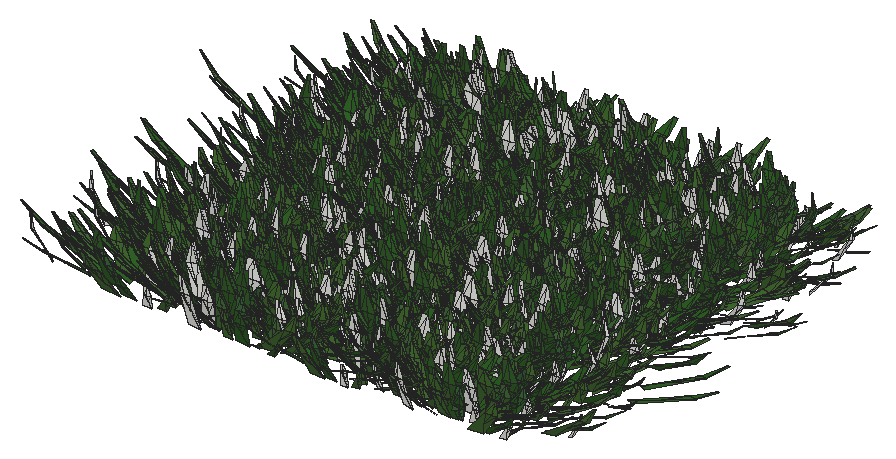
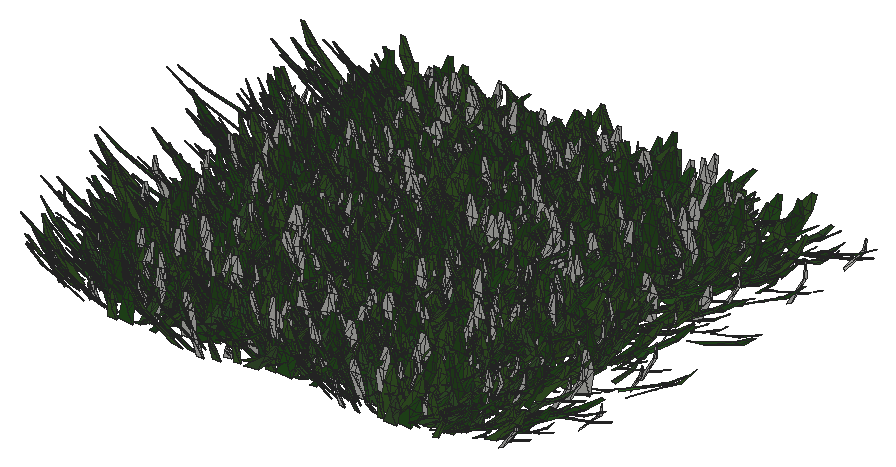
# SketchUp Ruby script. Lengths in inches.
U = 1.inch
M = Sketchup.active_model
def pt(a) = Geom::Point3d.new(a.map { |v| v * U })
def face(e, loops, mat)
  f = e.add_face(loops[0].map { |a| pt(a) })
  loops[1..].each { |l| e.add_face(l.map { |a| pt(a) }).erase! }
  f.material = f.back_material = mat if mat
  f
end
# faces: each face lists its corners as indices into pts; further lists are holes
def faces(e, pts, list, mat = nil) = list.each { |f| face(e, (f[0].is_a?(Array) ? f : [f]).map { |l| l.map { |i| pts[i] } }, mat) }
# xy, xz, yz: faces in a plane at the given z, y or x. An outline is a flat list of corners, or four numbers for a rectangle; further outlines are holes
def ring(l) = l.size == 4 ? [[l[0], l[1]], [l[2], l[1]], [l[2], l[3]], [l[0], l[3]]] : l.each_slice(2).to_a
def flat(e, list, mat, &to3) = list.each { |f| face(e, (f[0].is_a?(Array) ? f : [f]).map { |l| ring(l).map { |u, v| to3.(u, v) } }, mat) }
def xy(e, z, list, mat = nil) = flat(e, list, mat) { |x, y| [x, y, z] }
def xz(e, y, list, mat = nil) = flat(e, list, mat) { |x, z| [x, y, z] }
def yz(e, x, list, mat = nil) = flat(e, list, mat) { |y, z| [x, y, z] }
def lines(e, pts, list) = list.each { |a, b| e.add_line(pt(pts[a]), pt(pts[b])) }
# prism: a flat outline (further loops are holes) pulled along v
def prism(e, loops, v, mat = nil)
  f = face(e, loops, mat); d = Geom::Vector3d.new(v.map { |x| x * U })
  f.pushpull(f.normal.samedirection?(d) ? d.length : -d.length)
end
def box(e, o, s, mat = nil) = prism(e, [[o, [o[0] + s[0], o[1], o[2]], [o[0] + s[0], o[1] + s[1], o[2]], [o[0], o[1] + s[1], o[2]]]], [0, 0, s[2]], mat)
def at(x, y, z, deg = 0) = Geom::Transformation.translation(pt([x, y, z])) * Geom::Transformation.rotation(ORIGIN, Z_AXIS, deg.degrees)
def axes(o, x, y, z) = Geom::Transformation.new([*x, 0, *y, 0, *z, 0, *pt(o).to_a, 1])
def part(name) = M.definitions.add(name)
# library, detail: a bought-in or finely detailed component or shape, given as its bounding box
def library(name, o, s) = part(name).tap { |d| box(d.entities, o, s) }
def detail(e, o, s) = box(e.add_group.entities, o, s)
def put(e, d, t, mat = nil) = e.add_instance(d, t).tap { |i| i.material = mat if mat }
def group(e, t, mat = nil) = e.add_group.tap { |g| g.transformation = t; g.material = mat if mat }.entities
root = M.entities
M.materials.add("Material10").color = [48, 100, 38]
M.materials.add("Material3").color = [68, 110, 58]
M.materials.add("Material4").color = [48, 90, 38]
M.materials.add("Material5").color = [68, 110, 48]
M.materials.add("Material6").color = [48, 90, 48]
M.materials.add("Material7").color = [58, 110, 58]
M.materials.add("Material8").color = [58, 90, 38]
M.materials.add("Material9").color = [68, 100, 58]
c1 = part("grass00")
p = [[-0.6875,0.15,0],[-0.56,0.08,5.52],[-0.04,0.03,2.76],[0.48,-0.02,0],[0.35,-0.02,5.52],[-0.1,-0.14,5.52],
  [-0.12,0.65,8.37],[-0.42,0.65,8.37]]
faces(c1.entities,p,[[0,1,2,3],[3,2,4],[1,5,2],[5,4,2],[1,6,5],[4,5,6],[7,6,1]])
c2 = part("Group16\#1")
put(c2.entities,c1,axes([1.44,-0.61,-0.01],[0.05352,0.12609,0],[-0.10704,0.04543,0.07239],[0.06664,-0.02828,0.11628]),"Material6")
put(c2.entities,c1,axes([0.76,-0.15,-0.01],[0.04676,0.24062,0],[-0.23162,0.04501,0.06642],[0.0652,-0.01267,0.23595]),"Material3")
put(c2.entities,c1,axes([0.79,0.01,-0.01],[-0.00606,0.34651,0],[-0.34381,-0.00602,0.0432],[0.04319,0.00076,0.34386]))
put(c2.entities,c1,axes([1,0.23,-0.01],[-0.07192,0.31144,0],[-0.28722,-0.06632,0.1236],[0.12043,0.02781,0.29478]),"Material5")
put(c2.entities,c1,axes([1.66,0.77,-0.01],[-0.13828,0.29651,0],[-0.21551,-0.1005,0.22471],[0.20365,0.09498,0.23779]),"Material10")
put(c2.entities,c1,axes([0.6875,0.52,-0.01],[-0.18126,0.24051,0],[-0.22746,-0.17142,0.09788],[0.07817,0.05891,0.28481]),"Material5")
put(c2.entities,c1,axes([0.68,0.78,-0.01],[-0.215,0.18688,0],[-0.12385,-0.14248,0.21334],[0.13995,0.16101,0.18878]),"Material3")
put(c2.entities,c1,axes([0.56,1,-0.01],[-0.13756,0.07624,0],[-0.06159,-0.11112,0.0927],[0.04494,0.08108,0.12705]),"Material5")
put(c2.entities,c1,axes([0.2,0.64,-0.01],[-0.23729,0.07254,0],[-0.05711,-0.18681,0.153],[0.04473,0.14632,0.19535]),"Material10")
put(c2.entities,c1,axes([0.0625,0.72,-0.01],[-0.28874,0.02525,0],[-0.02179,-0.24916,0.14647],[0.01276,0.14591,0.25012]),"Material3")
put(c2.entities,c1,axes([-0.08,0.62,-0.01],[-0.34089,-0.04187,0],[0.03255,-0.26504,0.216],[-0.02633,0.21439,0.26703]),"Material10")
put(c2.entities,c1,axes([-0.34,0.98,-0.01],[-0.14314,-0.0493,0],[0.04397,-0.12769,0.06843],[-0.02228,0.0647,0.13505]),"Material10")
put(c2.entities,c1,axes([-0.87,1.45,-0.01],[-0.23488,-0.14114,0],[0.13761,-0.22901,0.06087],[-0.03135,0.05217,0.26717]))
put(c2.entities,c1,axes([-0.72,0.77,-0.01],[-0.14208,-0.13251,0],[0.07209,-0.0773,0.16301],[-0.11118,0.11922,0.1057]),"Material10")
put(c2.entities,c1,axes([-0.62,0.43,-0.01],[-0.14845,-0.21203,0],[0.18654,-0.13061,0.12304],[-0.10079,0.07057,0.22772]),"Material3")
put(c2.entities,c1,axes([-0.68,0.29,-0.01],[-0.13639,-0.32136,0],[0.31723,-0.13464,0.05579],[-0.05136,0.0218,0.34462]),"Material4")
put(c2.entities,c1,axes([-0.64,0.125,-0.01],[-0.0458,-0.23569,0],[0.22124,-0.043,0.08276],[-0.08124,0.01579,0.22538]),"Material7")
put(c2.entities,c1,axes([-1.6,-0.03,-0.01],[0.00576,-0.32897,0],[0.27526,0.00482,0.18018],[-0.18015,-0.00315,0.2753]),"Material5")
put(c2.entities,c1,axes([-1.36,-0.31,-0.01],[0.05718,-0.24765,0],[0.18172,0.04196,0.17267],[-0.16825,-0.03885,0.1865]),"Material10")
put(c2.entities,c1,axes([-1.54,-0.72,-0.01],[0.06537,-0.14017,0],[0.13555,0.06321,0.03939],[-0.0357,-0.01665,0.14956]))
put(c2.entities,c1,axes([-1.19,-0.9,-0.01],[0.09597,-0.12735,0],[0.11214,0.08451,0.07557],[-0.06035,-0.04548,0.14042]),"Material9")
put(c2.entities,c1,axes([-0.47,-0.54,-0.01],[0.11588,-0.10072,0],[0.0618,0.0711,0.12124],[-0.07953,-0.0915,0.0942]))
put(c2.entities,c1,axes([-0.47,-0.84,-0.01],[0.11927,-0.0661,0],[0.06603,0.11913,0.00646],[-0.00313,-0.00565,0.13621]),"Material5")
put(c2.entities,c1,axes([-0.38,-1.24,-0.01],[0.28037,-0.08571,0],[0.0618,0.20215,0.20315],[-0.05939,-0.19428,0.21139]),"Material9")
put(c2.entities,c1,axes([-0.06,-0.66,-0.01],[0.22719,-0.01987,0],[0.01247,0.14255,0.17758],[-0.01547,-0.17691,0.1431]),"Material8")
put(c2.entities,c1,axes([0.11,-0.89,-0.01],[0.14882,0.01828,0],[-0.01058,0.08611,0.12229],[0.01491,-0.12138,0.08676]),"Material6")
put(c2.entities,c1,axes([0.25,-0.72,-0.01],[0.20481,0.07053,0],[-0.06206,0.18022,0.10291],[0.03351,-0.0973,0.1906]),"Material6")
put(c2.entities,c1,axes([0.85,-1.42,-0.01],[0.16481,0.09904,0],[-0.09472,0.15762,0.05616],[0.02893,-0.04814,0.18389]),"Material5")
put(c2.entities,c1,axes([1.01,-1.09,-0.01],[0.21858,0.20385,0],[-0.17495,0.1876,0.15339],[0.10462,-0.11218,0.25652]),"Material10")
put(c2.entities,c1,axes([1.01,-0.71,-0.01],[0.08733,0.12473,0],[-0.06445,0.04512,0.13037],[0.1068,-0.07477,0.07867]),"Material6")
c3 = part("Group15\#1")
put(c3.entities,c2,at(0,0,0))
c4 = part("3darcstudiotree_grass00\#1")
put(c4.entities,c3,at(0,0,0))
put(root,c4,axes([993.125,915.59,0],[-3.60582,-0.24196,0],[1.04886,-0.97693,-0.03217],[0.06139,-0.05718,1.86146]))
put(root,c4,axes([991.19,900.47,0],[2.28978,0.96186,0],[-3.76338,0.55994,-0.00188],[-0.01111,0.00165,1.87843]))
put(root,c4,axes([991.63,916.75,0],[2.13866,0.74246,0],[-3.14038,0.56537,-0.02117],[-0.12042,0.02168,1.69559]))
put(root,c4,axes([992.37,908.81,0],[-2.16053,0.9205,0],[-4.3515,-0.63835,-0.01374],[-0.05636,-0.00827,1.50009]))
put(root,c4,axes([991.97,894.3,0],[0.82896,1.15167,0],[-5.08245,0.22864,-0.03105],[-0.14233,0.0064,1.50318]))
put(root,c4,axes([992.18,919.85,0],[4.96916,0.09392,0],[-0.36542,1.20834,-0.04634],[-0.02294,0.07584,1.98901]))
put(root,c4,axes([992.33,926.2,0],[1.48031,1.01744,0],[-4.79783,0.43628,-0.0524],[-0.2112,0.01921,1.36852]))
put(root,c4,axes([994.4,929.09,0],[-4.63446,-0.46393,0],[1.56749,-0.97866,-0.04264],[0.10164,-0.06346,1.69007]))
put(root,c4,axes([993.33,930.77,0],[3.16295,-0.50135,0],[2.10496,0.83,-0.03299],[0.1278,0.05039,1.77748]))
put(root,c4,axes([993.96,903.53,0],[-3.25579,0.4273,0],[-2.23495,-1.06431,-0.02543],[-0.07509,-0.03576,1.9093]))
put(root,c4,axes([993.17,931.78,0],[2.11626,0.74991,0],[-2.96839,0.52355,-0.03223],[-0.15972,0.02817,1.37708]))
put(root,c4,axes([993.58,904.93,0],[2.21507,0.97624,0],[-3.15725,0.44774,-0.03898],[-0.29704,0.04212,1.98748]))
put(root,c4,axes([993.98,924.32,0],[2.51481,0.74573,0],[-2.81558,0.59343,-0.04117],[-0.21226,0.04474,1.55213]))
put(root,c4,axes([993.95,898.47,0],[0.22886,1.14034,0],[-4.67986,0.0587,-0.03261],[-0.20676,0.00259,1.85888]))
put(root,c4,axes([993.79,912.43,0],[1.19223,1.00137,0],[-3.72637,0.27729,-0.00785],[-0.05882,0.00438,1.89978]))
put(root,c4,axes([994.03,923.01,0],[2.95745,0.80625,0],[-2.67106,0.61236,-0.03804],[-0.21785,0.04994,1.7602]))
put(root,c4,axes([996.94,916.93,0],[-2.68493,-0.72179,0],[2.74212,-0.63751,-0.03633],[0.19715,-0.04583,1.73438]))
put(root,c4,axes([997.05,915.26,0],[-1.94469,-0.81082,0],[3.41072,-0.51128,-0.04451],[0.23926,-0.03587,1.55797]))
put(root,c4,axes([997.6,907.85,0],[-4.38536,-0.48819,0],[1.68539,-0.94622,-0.04343],[0.09225,-0.05179,1.35201]))
put(root,c4,axes([997.3125,903.34,0],[-0.93763,-1.01509,0],[3.58265,-0.20683,-0.0292],[0.19066,-0.01101,1.53984]))
put(root,c4,axes([997.54,933.23,0],[-2.99891,-0.51884,0],[2.25803,-0.81571,-0.03348],[0.14398,-0.05201,1.87437]))
put(root,c4,axes([997.02,908.78,0],[2.32628,-1.10135,0],[3.26689,0.43127,-0.03491],[0.22091,0.02916,1.65255]))
put(root,c4,axes([997.82,895.31,0],[-3.78007,0.18751,0],[-0.9942,-1.25267,-0.05548],[-0.05563,-0.0701,1.6451]))
put(root,c4,axes([999.06,923.07,0],[-3.41877,-0.81095,0],[3.11222,-0.82002,-0.00166],[0.00704,-0.00186,1.74215]))
put(root,c4,axes([997.04,927.79,0],[3.56011,0.3766,0],[-1.5529,0.91751,-0.02719],[-0.08207,0.04849,1.929]))
put(root,c4,axes([997.06,928.26,0],[-0.28146,1.0454,0],[-4.85505,-0.0817,-0.01753],[-0.10805,-0.00182,1.87889]))
put(root,c4,axes([996.96,913.24,0],[4.34869,0.47354,0],[-1.70545,0.97885,-0.04191],[-0.08317,0.04774,1.32656]))
put(root,c4,axes([997.59,932.22,0],[0.50605,0.98572,0],[-4.41784,0.14175,-0.0516],[-0.36721,0.01178,1.99718]))
put(root,c4,axes([997.4,919.9375,0],[4.51798,0.20316,0],[-0.79252,1.10155,-0.03729],[-0.03789,0.05267,1.60628]))
put(root,c4,axes([999.3125,901.25,0],[-4.34417,-0.18262,0],[0.70687,-1.05094,-0.0114],[0.01401,-0.02082,1.97478]))
put(root,c4,axes([997.67,917.93,0],[2.21014,1.15532,0],[-3.78234,0.45223,-0.02212],[-0.14871,0.01778,1.95299]))
put(root,c4,axes([997.98,906.54,0],[-0.29005,1.03921,0],[-4.26068,-0.07432,-0.02357],[-0.13601,-0.00237,1.54387]))
put(root,c4,axes([997.99,899.8,0],[4.64548,-0.02052,0],[0.0884,1.25077,-0.02875],[0.00253,0.03584,1.55972]))
put(root,c4,axes([998.15,924.42,0],[2.69774,0.60172,0],[-2.53829,0.71125,-0.00625],[-0.03018,0.00846,1.72796]))
put(root,c4,axes([999.74,911.61,0],[-4.15604,0.63305,0],[-2.33124,-0.95655,-0.05764],[-0.19304,-0.07921,1.8024]))
put(root,c4,axes([1000.16,896.98,0],[1.24811,-0.98204,0],[4.93225,0.39179,-0.03698],[0.19941,0.01584,1.82987]))
put(root,c4,axes([1000.78,904.14,0],[-2.73285,-0.87798,0],[3.13409,-0.60971,-0.01663],[0.09994,-0.01944,1.89037]))
put(root,c4,axes([1000.38,894.13,0],[-3.26487,0.7652,0],[-2.88539,-0.76944,-0.04557],[-0.23173,-0.0618,1.96028]))
put(root,c4,axes([999.96,920.85,0],[-2.34155,0.84913,0],[-3.4682,-0.59774,-0.02321],[-0.12342,-0.02127,1.70026]))
put(root,c4,axes([1000.68,899.02,0],[-3.68799,0.26675,0],[-1.34322,-1.16069,-0.00573],[-0.00843,-0.00729,1.59925]))
put(root,c4,axes([1000.62,926.1,0],[2.33049,-0.73294,0],[3.96124,0.7872,-0.06111],[0.26943,0.05354,1.78135]))
put(root,c4,axes([1000.74,930.75,0],[3.80611,-0.44418,0],[1.98468,1.06289,-0.02938],[0.0699,0.03743,1.64954]))
put(root,c4,axes([1000.54,910.75,0],[5.11514,-0.08131,0],[0.26106,1.02638,-0.03177],[0.01497,0.05885,1.90853]))
put(root,c4,axes([1002.97,915.48,0],[-4.00581,-0.59681,0],[2.18474,-0.9165,-0.01663],[0.06212,-0.02606,1.94585]))
put(root,c4,axes([1003.13,894.17,0],[3.537,-0.94689,0],[2.76209,0.64485,-0.01281],[0.06208,0.01449,1.56626]))
put(root,c4,axes([1004.74,912.09,0],[-1.77,-0.83286,0],[4.02387,-0.53447,-0.00698],[0.04087,-0.00543,1.8873]))
put(root,c4,axes([1004.35,896.8,0],[1.67638,-1.0425,0],[4.59893,0.4622,-0.01772],[0.09487,0.00953,1.7874]))
put(root,c4,axes([1004.92,903.24,0],[-3.4263,-0.91381,0],[3.1573,-0.73989,-0.03051],[0.13581,-0.03183,1.65027]))
put(root,c4,axes([1004.25,929.875,0],[2.30637,-1.06411,0],[3.89478,0.5276,-0.00988],[0.05923,0.00802,1.88737]))
put(root,c4,axes([1003.125,907.38,0],[5.17876,0.00972,0],[-0.03633,1.20929,-0.012],[-0.00051,0.01694,1.70791]))
put(root,c4,axes([1003.94,895.44,0],[3.44483,-0.53348,0],[2.02838,0.81862,-0.00486],[0.01517,0.00612,1.42853]))
put(root,c4,axes([1003.27,909.05,0],[1.61317,1.05687,0],[-3.89248,0.37133,-0.03212],[-0.19954,0.01904,1.73128]))
put(root,c4,axes([1003.67,899.93,0],[4.23132,0.05428,0],[-0.26252,1.27912,-0.05168],[-0.01396,0.06804,1.68853]))
put(root,c4,axes([1003.49,904.64,0],[0.18775,1.28338,0],[-5.04354,0.04611,-0.0182],[-0.08343,0.00076,1.44668]))
put(root,c4,axes([1003.66,917.75,0],[0.66659,0.99759,0],[-3.70369,0.15468,-0.00028],[-0.00179,0.00007,1.50491]))
put(root,c4,axes([1004.01,928.82,0],[-0.12653,1.00906,0],[-4.40907,-0.03456,-0.04067],[-0.22619,-0.00177,1.53414]))
put(root,c4,axes([1004.9,922.97,0],[-3.44749,0.85218,0],[-2.82175,-0.71346,-0.03762],[-0.15511,-0.03922,1.47105]))
put(root,c4,axes([1003.65,926.27,0],[0.53467,1.10303,0],[-5.00046,0.15149,-0.01569],[-0.0735,0.00223,1.48562]))
put(root,c4,axes([1006.01,919.96,0],[-3.66347,-0.90665,0],[3.59625,-0.9082,-0.03717],[0.1584,-0.04,1.93537]))
put(root,c4,axes([1005.79,916.38,0],[-4.4143,-0.18542,0],[0.67487,-1.00419,-0.01654],[0.02043,-0.03039,1.89711]))
put(root,c4,axes([1006.22,920.95,0],[-1.79213,-0.89815,0],[3.71156,-0.46287,-0.00448],[0.02956,-0.00369,1.90991]))
put(root,c4,axes([1005.32,906.62,0],[-3.49749,0.50247,0],[-2.5408,-1.10534,-0.04948],[-0.12396,-0.05393,1.60238]))
put(root,c4,axes([1004.72,924.46,0],[0.73607,0.9032,0],[-4.03456,0.2055,-0.04728],[-0.29589,0.01507,1.64346]))
put(root,c4,axes([1005.08,913.52,0],[3.54729,0.43846,0],[-1.7678,0.89387,-0.03066],[-0.09543,0.04825,1.75054]))
put(root,c4,axes([1006.28,898.99,0],[0.42302,-0.9917,0],[3.83549,0.10225,-0.04937],[0.35058,0.00935,1.72169]))
put(root,c4,axes([1006.54,910.39,0],[-1.77196,1.05602,0],[-3.98674,-0.4181,-0.04701],[-0.29505,-0.03094,1.83905]))
put(root,c4,axes([1006.75,901.58,0],[0.45093,1.12107,0],[-3.84241,0.0966,-0.04963],[-0.30261,0.00761,1.47912]))
put(root,c4,axes([1006.0625,931.48,0],[3.32772,0.78374,0],[-3.41591,0.90649,-0.01047],[-0.04436,0.01177,1.92288]))
put(root,c4,axes([1007.19,926.93,0],[4.23567,0.36269,0],[-1.24548,0.90909,-0.02009],[-0.04731,0.03453,1.7458]))
put(root,c4,axes([1009.07,926.16,0],[-4.4227,-0.30365,0],[1.03811,-0.94502,-0.02848],[0.05651,-0.05144,1.83531]))
put(root,c4,axes([1008.78,930.36,0],[-0.43672,-1.24202,0],[4.36716,-0.09597,-0.04765],[0.30496,-0.0067,1.76037]))
put(root,c4,axes([1009.02,932.1,0],[-4.11211,0.64037,0],[-1.92557,-0.77282,-0.01072],[-0.04599,-0.01846,1.84718]))
put(root,c4,axes([1009.62,904.5,0],[-4.34593,0.58001,0],[-2.21528,-1.03742,-0.03463],[-0.1032,-0.04833,1.86049]))
put(root,c4,axes([1009.16,909.29,0],[-1.86227,1.06204,0],[-3.42788,-0.37567,-0.01229],[-0.09526,-0.01044,1.9803]))
put(root,c4,axes([1010.71,924.18,0],[-3.5926,-0.75101,0],[3.19063,-0.95393,-0.04137],[0.11689,-0.03495,1.36909]))
put(root,c4,axes([1010.18,918.31,0],[3.48166,-0.50059,0],[2.44605,1.06327,-0.03788],[0.08627,0.0375,1.40078]))
put(root,c4,axes([1009.55,916.45,0],[4.43547,0.23328,0],[-0.86743,1.0308,-0.04482],[-0.053,0.06298,1.51278]))
put(root,c4,axes([1011.49,927.04,0],[-3.11664,-0.68281,0],[2.49826,-0.71269,-0.01406],[0.06937,-0.01979,1.77353]))
put(root,c4,axes([1010.57,922.89,0],[4.18182,-0.37358,0],[1.54336,1.07977,-0.0155],[0.03636,0.02544,1.9985]))
put(root,c4,axes([1012.02,900.56,0],[-2.65841,-0.80925,0],[2.97739,-0.6113,-0.021],[0.09455,-0.01941,1.40308]))
put(root,c4,axes([1011.95,905.66,0],[-1.89766,-0.97867,0],[3.50817,-0.42515,-0.03263],[0.22536,-0.02731,1.87]))
put(root,c4,axes([1010.76,921.43,0],[3.92204,-0.31031,0],[1.16336,0.91899,-0.04021],[0.0777,0.06138,1.5432]))
put(root,c4,axes([1012.13,903.57,0],[-4.71443,0.13943,0],[-0.55237,-1.16732,-0.02284],[-0.01323,-0.02795,1.44864]))
put(root,c4,axes([1011.54,898.25,0],[-2.39721,0.74853,0],[-3.19848,-0.64021,-0.02462],[-0.14683,-0.02939,1.95656]))
put(root,c4,axes([1010.91,895.96,0],[3.23025,0.97107,0],[-3.57979,0.74426,-0.02991],[-0.15449,0.03212,1.95467]))
put(root,c4,axes([1012.86,933.43,0],[-2.21429,-1.09214,0],[3.31642,-0.42025,-0.03791],[0.27447,-0.03478,1.88609]))
put(root,c4,axes([1012.94,910.82,0],[0.02853,-0.96411,0],[5.08808,0.00941,-0.04606],[0.26224,0.00049,1.81052]))
put(root,c4,axes([1011.22,912.01,0],[3.66614,0.51192,0],[-1.98914,0.89033,-0.02091],[-0.0622,0.02784,1.55496]))
put(root,c4,axes([1011.11,919.75,0],[4.6069,0.58631,0],[-2.28752,1.12337,-0.01612],[-0.03759,0.01846,1.61949]))
put(root,c4,axes([1012.7,914.1,0],[-3.88433,0.51238,0],[-1.98517,-0.9406,-0.01893],[-0.04557,-0.02159,1.37131]))
put(root,c4,axes([1012.73,897.33,0],[-3.68297,0.59369,0],[-2.11941,-0.82173,-0.01497],[-0.04852,-0.01881,1.4615]))
put(root,c4,axes([1012.04,894,0],[0.49612,1.17734,0],[-3.69255,0.09725,-0.01763],[-0.12152,0.0032,1.60818]))
put(root,c4,axes([1012.29,915.04,0],[3.11929,0.72453,0],[-2.48773,0.6694,-0.03885],[-0.22621,0.06087,1.95422]))
put(root,c4,axes([1012.86,928.59,0],[3.97995,-0.28298,0],[1.30466,1.14685,-0.03545],[0.05768,0.0507,1.77295]))
put(root,c4,axes([1012.54,907.52,0],[0.95512,1.24392,0],[-4.78219,0.22949,-0.02457],[-0.12659,0.00607,1.59681]))
put(root,c4,axes([1013.17,901.16,0],[4.18474,0.7675,0],[-2.60572,0.88797,-0.00415],[-0.01182,0.00403,1.32509]))
put(root,c4,axes([1014.85,904.92,0],[1.49904,-0.99382,0],[4.36571,0.41157,-0.04892],[0.30393,0.02865,1.93615]))
put(root,c4,axes([1015.58,918.22,0],[-3.34703,-0.44034,0],[1.86344,-0.88525,-0.01604],[0.05682,-0.02699,1.9024]))
put(root,c4,axes([1015.74,924.29,0],[-0.87549,-1.06671,0],[4.68602,-0.24038,-0.03341],[0.20374,-0.01045,1.86102]))
put(root,c4,axes([1015.35,903.09,0],[1.68499,-1.00901,0],[4.65536,0.48589,-0.03949],[0.20736,0.02164,1.7941]))
put(root,c4,axes([1016.07,912.65,0],[-2.77219,-0.80321,0],[3.53234,-0.76197,-0.03179],[0.10998,-0.02372,1.33245]))
put(root,c4,axes([1016.625,920.68,0],[0.45917,-1.01545,0],[5.11405,0.14453,-0.01256],[0.07404,0.00209,1.90836]))
put(root,c4,axes([1014.95,897.43,0],[3.91432,0.2962,0],[-1.14145,0.94277,-0.0422],[-0.0933,0.07706,1.87907]))
put(root,c4,axes([1015.41,913.11,0],[4.97696,-0.05302,0],[0.19507,1.14438,-0.04096],[0.01048,0.0615,1.72127]))
put(root,c4,axes([1017.36,907.75,0],[-1.27908,-0.88935,0],[3.91716,-0.35211,-0.0171],[0.11094,-0.00997,1.79343]))
put(root,c4,axes([1016.96,930.41,0],[-4.79032,0.48606,0],[-1.70961,-1.05304,-0.01879],[-0.03655,-0.02252,1.46955]))
put(root,c4,axes([1017.31,901.75,0],[-3.54874,-0.19762,0],[0.84752,-0.95118,-0.02543],[0.03659,-0.04107,1.61262]))
put(root,c4,axes([1016.69,922.97,0],[-3.16014,0.66861,0],[-3.08586,-0.91157,-0.05904],[-0.18903,-0.05584,1.47981]))
put(root,c4,axes([1017.54,899.93,0],[1.28054,-1.03018,0],[4.2523,0.33036,-0.02169],[0.11477,0.00892,1.54236]))
put(root,c4,axes([1018.04,897.93,0],[-0.71824,-1.02023,0],[5.03908,-0.22172,-0.05842],[0.35675,-0.0157,1.98292]))
put(root,c4,axes([1017.16,915.72,0],[4.32394,-0.4782,0],[1.59071,0.89896,-0.00969],[0.0217,0.01226,1.36001]))
put(root,c4,axes([1018.625,910.32,0],[-4.09477,-0.54974,0],[1.8737,-0.87227,-0.0264],[0.09985,-0.04648,1.979]))
put(root,c4,axes([1018.46,928.35,0],[-4.29836,-0.05077,0],[0.23538,-1.24557,-0.03065],[0.00914,-0.04835,1.9691]))
put(root,c4,axes([1016.7,917.06,0],[4.80121,0.29914,0],[-1.24856,1.25248,-0.03274],[-0.0398,0.03992,1.62193]))
put(root,c4,axes([1018.79,906.04,0],[-3.91367,-0.4767,0],[2.06304,-1.05859,-0.02869],[0.08103,-0.04158,1.89824]))
put(root,c4,axes([1017.14,908.58,0],[4.81743,-0.02087,0],[0.06672,0.96257,-0.04649],[0.00527,0.07597,1.57333]))
put(root,c4,axes([1017.97,931.61,0],[4.37292,-0.40538,0],[1.54259,1.04001,-0.01564],[0.037,0.02495,1.88746]))
put(root,c4,axes([1018.09,926.71,0],[-1.42316,0.86255,0],[-3.977,-0.41012,-0.01866],[-0.09986,-0.0103,1.55626]))
put(root,c4,axes([1018.75,919.49,0],[5.06053,-0.0101,0],[0.03814,1.19402,-0.00522],[0.0002,0.00625,1.42947]))
put(root,c4,axes([1018.96,925.47,0],[1.90816,0.82105,0],[-3.58285,0.52042,-0.03711],[-0.20984,0.03048,1.69359]))
put(root,c4,axes([1018.79,895.0625,0],[2.85091,0.72979,0],[-2.82823,0.69053,-0.01838],[-0.08823,0.02154,1.65818]))
put(root,c4,axes([1021.12,909.27,0],[-4.57395,-0.56919,0],[2.24978,-1.12995,-0.0574],[0.11462,-0.05757,1.41402]))
put(root,c4,axes([1021.47,930.0625,0],[-4.36386,0.0424,0],[-0.14663,-0.94321,-0.04521],[-0.01421,-0.09143,1.91035]))
put(root,c4,axes([1021.95,922.82,0],[-3.84808,-0.62814,0],[2.34387,-0.89743,-0.0556],[0.18939,-0.07251,1.66946]))
put(root,c4,axes([1020.91,913.97,0],[-2.81015,0.82442,0],[-3.69627,-0.78745,-0.01912],[-0.06485,-0.01382,1.35238]))
put(root,c4,axes([1022.22,901.24,0],[-3.5015,-0.36139,0],[1.44415,-0.87453,-0.01181],[0.03303,-0.02,1.73426]))
put(root,c4,axes([1022.05,907.67,0],[-0.56459,-1.01387,0],[4.32656,-0.15058,-0.04493],[0.31224,-0.01087,1.91565]))
put(root,c4,axes([1022.15,928.47,0],[0.89168,-0.93114,0],[3.99265,0.23897,-0.00366],[0.02101,0.00126,1.51551]))
put(root,c4,axes([1022.73,900.5625,0],[0.23484,-1.14494,0],[3.96232,0.0508,-0.01161],[0.06761,0.00087,1.44612]))
put(root,c4,axes([1023.41,918.68,0],[-3.5181,-0.78299,0],[2.9623,-0.83188,-0.03256],[0.12635,-0.03548,1.62483]))
put(root,c4,axes([1022.9,933.21,0],[-3.45708,0.57656,0],[-2.12905,-0.79787,-0.03251],[-0.13485,-0.05053,1.79208]))
put(root,c4,axes([1023.5,921.57,0],[-3.94189,0.10624,0],[-0.456,-1.0575,-0.01956],[-0.01557,-0.0361,1.97453]))
put(root,c4,axes([1022.12,895.54,0],[-0.1159,1.07064,0],[-4.16097,-0.02815,-0.00627],[-0.03911,-0.00026,1.62459]))
put(root,c4,axes([1024.0625,931.47,0],[-2.63935,-0.88257,0],[3.19573,-0.59731,-0.02089],[0.10644,-0.01989,1.58683]))
put(root,c4,axes([1023.38,904.63,0],[-3.39832,0.86181,0],[-2.85508,-0.70364,-0.05097],[-0.26206,-0.06459,1.80901]))
put(root,c4,axes([1022.97,894.2,0],[-2.0463,0.79301,0],[-3.44855,-0.55617,-0.00439],[-0.02397,-0.00387,1.66469]))
put(root,c4,axes([1022.94,927.27,0],[-1.30702,1.14892,0],[-3.96735,-0.28208,-0.01558],[-0.11053,-0.00786,1.90128]))
put(root,c4,axes([1022.5,911.65,0],[3.62958,0.6733,0],[-2.52662,0.85126,-0.02502],[-0.10717,0.03611,1.90511]))
put(root,c4,axes([1024.74,925.72,0],[-1.1386,-0.97265,0],[4.79603,-0.3509,-0.04795],[0.2257,-0.01651,1.53186]))
put(root,c4,axes([1023.16,898.19,0],[-0.88584,1.09832,0],[-4.93295,-0.24867,-0.03197],[-0.17795,-0.00897,1.78572]))
put(root,c4,axes([1024.59,897.01,0],[-3.95588,0.56377,0],[-2.45949,-1.07862,-0.01918],[-0.05514,-0.02418,1.80194]))
put(root,c4,axes([1024.64,910.28,0],[1.93293,-0.87029,0],[3.69238,0.51255,-0.03203],[0.18787,0.02608,1.771]))
put(root,c4,axes([1024.52,924.75,0],[-3.12402,0.89295,0],[-3.68078,-0.80483,-0.03347],[-0.1578,-0.0345,1.91416]))
put(root,c4,axes([1023.9,905.53,0],[4.8764,0.03202,0],[-0.108,1.02786,-0.04419],[-0.00896,0.08526,1.98467]))
put(root,c4,axes([1025.38,919.6,0],[-4.39634,0.48093,0],[-1.83375,-1.04768,-0.02625],[-0.05381,-0.03075,1.46233]))
put(root,c4,axes([1024.52,914.82,0],[-0.42678,0.97311,0],[-4.0579,-0.11123,-0.02456],[-0.16336,-0.00448,1.70727]))
put(root,c4,axes([1024.47,902.92,0],[5.0854,0.12715,0],[-0.47106,1.17748,-0.02551],[-0.01271,0.03178,1.48132]))
put(root,c4,axes([1025.1,916.29,0],[3.65373,-0.31511,0],[1.20707,0.87477,-0.03311],[0.07347,0.05325,1.57439]))
